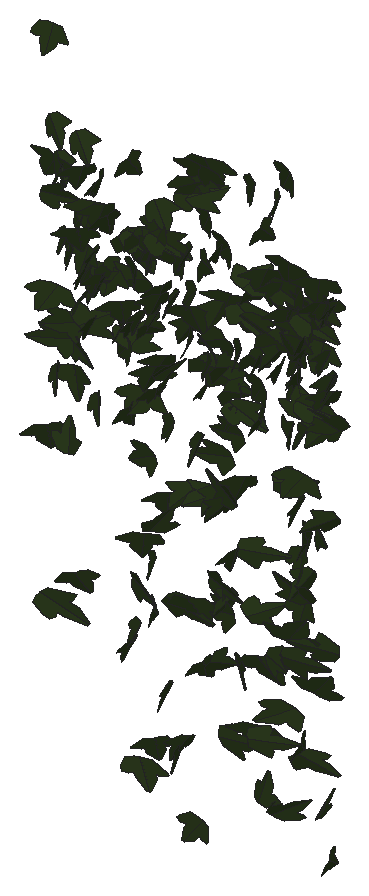
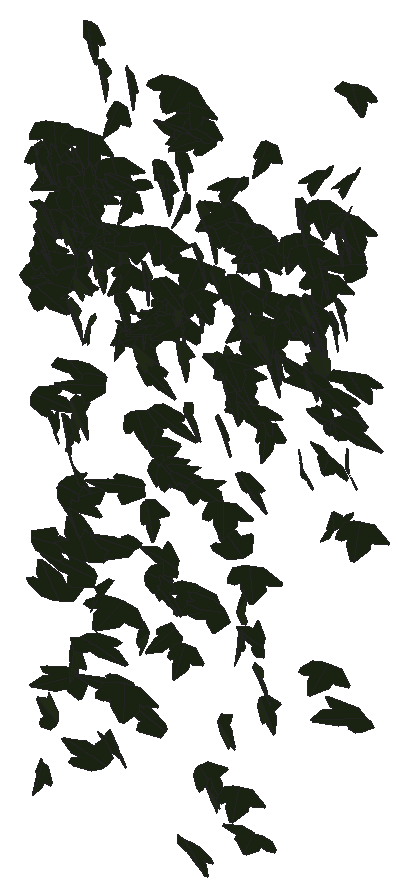
# SketchUp Ruby script. Lengths in millimetres.
U = 1.mm
M = Sketchup.active_model
def pt(a) = Geom::Point3d.new(a.map { |v| v * U })
def face(e, loops, mat)
  f = e.add_face(loops[0].map { |a| pt(a) })
  loops[1..].each { |l| e.add_face(l.map { |a| pt(a) }).erase! }
  f.material = f.back_material = mat if mat
  f
end
# faces: each face lists its corners as indices into pts; further lists are holes
def faces(e, pts, list, mat = nil) = list.each { |f| face(e, (f[0].is_a?(Array) ? f : [f]).map { |l| l.map { |i| pts[i] } }, mat) }
# xy, xz, yz: faces in a plane at the given z, y or x. An outline is a flat list of corners, or four numbers for a rectangle; further outlines are holes
def ring(l) = l.size == 4 ? [[l[0], l[1]], [l[2], l[1]], [l[2], l[3]], [l[0], l[3]]] : l.each_slice(2).to_a
def flat(e, list, mat, &to3) = list.each { |f| face(e, (f[0].is_a?(Array) ? f : [f]).map { |l| ring(l).map { |u, v| to3.(u, v) } }, mat) }
def xy(e, z, list, mat = nil) = flat(e, list, mat) { |x, y| [x, y, z] }
def xz(e, y, list, mat = nil) = flat(e, list, mat) { |x, z| [x, y, z] }
def yz(e, x, list, mat = nil) = flat(e, list, mat) { |y, z| [x, y, z] }
def lines(e, pts, list) = list.each { |a, b| e.add_line(pt(pts[a]), pt(pts[b])) }
# prism: a flat outline (further loops are holes) pulled along v
def prism(e, loops, v, mat = nil)
  f = face(e, loops, mat); d = Geom::Vector3d.new(v.map { |x| x * U })
  f.pushpull(f.normal.samedirection?(d) ? d.length : -d.length)
end
def box(e, o, s, mat = nil) = prism(e, [[o, [o[0] + s[0], o[1], o[2]], [o[0] + s[0], o[1] + s[1], o[2]], [o[0], o[1] + s[1], o[2]]]], [0, 0, s[2]], mat)
def at(x, y, z, deg = 0) = Geom::Transformation.translation(pt([x, y, z])) * Geom::Transformation.rotation(ORIGIN, Z_AXIS, deg.degrees)
def axes(o, x, y, z) = Geom::Transformation.new([*x, 0, *y, 0, *z, 0, *pt(o).to_a, 1])
def part(name) = M.definitions.add(name)
# library, detail: a bought-in or finely detailed component or shape, given as its bounding box
def library(name, o, s) = part(name).tap { |d| box(d.entities, o, s) }
def detail(e, o, s) = box(e.add_group.entities, o, s)
def put(e, d, t, mat = nil) = e.add_instance(d, t).tap { |i| i.material = mat if mat }
def group(e, t, mat = nil) = e.add_group.tap { |g| g.transformation = t; g.material = mat if mat }.entities
root = M.entities
M.materials.add("efeu2").color = [43, 57, 29]
c1 = part("ivyleaf_10")
p = [[0,12.8,-0.8],[-1.5,51.3,-10.9],[-4.9,51,-11.6],[-13.6,26.5,-7.3],[-13.2,15.9,-4.6],[-21.1,19.3,-7.2],
  [-29.5,16.3,-8.3],[-29.2,8.3,-6.2],[-19.7,-9.8,0.5],[-7.6,-13,4],[1,-12.2,5.8],[-0.4,51.1,-11.1],
  [-1.5,51.1,-10.9],[1,-12.4,5.9],[16.9,-12.4,3.5],[35.1,9.1,-5.1],[35,12.9,-6.1],[20.5,16.4,-4.9],
  [15.8,15,-3.8],[15.3,27.6,-7.1],[12.8,31.3,-7.8]]
faces(c1.entities,p,[[0,1,2,3,4,5,6,7,8,9,10],[11,12,0,13,14,15,16,17,18,19,20]],"efeu2")
put(root,c1,axes([857.1,1048,494],[-0.76417,-0.56364,-0.16539],[0.1854,0.13367,-0.69203],[1.10248,-0.41316,0.00174]))
put(root,c1,axes([875.9,1057.8,630.2],[0.62914,-0.04984,-0.57145],[-1.07511,0.08633,-0.3343],[0.18971,0.65451,0.00058]))
put(root,c1,axes([856.2,1056.8,1082.8],[0.86369,0.09119,-0.06828],[-0.08573,0.01132,-0.71351],[-0.10938,0.71114,0.02012]))
put(root,c1,axes([872.4,1048.6,897.9],[-1.16361,0.05516,0.27789],[-0.53203,-0.01005,-0.61304],[-0.08762,-0.67151,0.032]))
put(root,c1,axes([862.5,1054.4,698],[1.15679,0.14069,-0.19865],[-0.37438,-0.03088,-0.62374],[-0.27291,0.63871,0.0136]))
put(root,c1,axes([862.7,1060,578.1],[0.46837,-0.34978,0.49712],[0.59384,-0.38757,-0.42716],[0.99279,0.39684,0.02098]))
put(root,c1,axes([875.6,1051.7,887.6],[0.36125,-0.62169,-0.15977],[-0.00089,0.16647,-0.64834],[1.22165,0.18396,0.04677]))
put(root,c1,axes([871.3,1044.2,956.8],[0.07417,0.6859,-0.01278],[-0.00011,-0.01279,-0.68701],[-1.30563,0.03897,-0.00067]))
put(root,c1,axes([891.2,1053.3,661.6],[0.80097,-0.16994,-0.48499],[-0.85913,0.17735,-0.45386],[0.46745,0.61716,-0.00312]))
put(root,c1,axes([862.4,1046.6,844.8],[0.22257,-0.09676,0.68328],[0.60747,0.5078,-0.06104],[-0.58293,0.49224,0.19728]))
put(root,c1,axes([879.6,1055.6,783],[0.43516,-0.59083,-0.12994],[-0.02273,0.13448,-0.63247],[1.15111,0.22601,0.03663]))
put(root,c1,axes([883.5,1054.5,881.1],[0.46084,-0.57742,-0.21843],[-0.01855,0.23103,-0.62152],[1.1748,0.23015,0.07587]))
put(root,c1,axes([879.2,1048,902.4],[0.0145,0.67002,-0.10036],[-0.00753,-0.10032,-0.67006],[-1.28939,0.00812,0.00278]))
put(root,c1,axes([889.4,1054.8,764.6],[0.41365,-0.53615,-0.27461],[-0.06271,0.28092,-0.57454],[1.14473,0.20913,0.06776]))
put(root,c1,axes([864.2,1046,242.4],[0.609,0.20168,0.61131],[1.00332,0.30965,-0.37811],[-0.70305,0.61661,-0.01007]))
put(root,c1,axes([894.2,1044.3,482.4],[0.22662,0.60555,-0.37945],[0.10475,0.37577,0.61695],[1.35602,-0.13023,0.01576]))
put(root,c1,axes([890.1,1061.3,582.8],[1.0221,-0.25445,0.29182],[0.52582,-0.09774,-0.59366],[0.51623,0.60334,0.0269]))
put(root,c1,axes([906.6,1054.5,828.8],[0.49026,-0.5364,-0.28712],[-0.1041,0.29012,-0.59107],[1.15324,0.25422,0.06871]))
put(root,c1,axes([906.8,1050.1,291.4],[-0.81787,-0.39488,-0.26374],[0.33783,0.19634,-0.58319],[0.83824,-0.46442,-0.0223]))
put(root,c1,axes([911.5,1045.7,805.6],[-0.88124,-0.45718,-0.09759],[0.11767,0.07626,-0.65061],[0.88189,-0.46702,-0.01071]))
put(root,c1,axes([913.5,1054.2,746.1],[0.28575,-0.62987,-0.03437],[-0.0113,0.03391,-0.64751],[1.2005,0.15024,0.00209]))
put(root,c1,axes([916,1046.3,899.7],[-0.52099,-0.60983,-0.01375],[0.00795,0.0132,-0.66845],[1.16089,-0.27377,-0.00159]))
put(root,c1,axes([907.1,1054.1,696.2],[-0.00905,-0.59614,-0.30589],[0.16466,-0.30388,0.59089],[-1.26454,-0.0353,0.07913]))
put(root,c1,axes([895.3,1055.6,628.7],[0.19219,-0.14159,0.61257],[1.06825,-0.25923,-0.15244],[0.53911,0.56413,0.08369]))
put(root,c1,axes([918.4,1053.9,750.5],[0.5931,-0.52045,-0.23254],[-0.09072,0.2403,-0.6017],[1.08109,0.30569,0.07708]))
put(root,c1,axes([913.6,1056,773.9],[1.02959,-0.36291,0.04755],[0.09164,-0.01356,-0.65125],[0.69055,0.5429,0.01552]))
put(root,c1,axes([915.3,1044.1,946.2],[0.22831,0.67336,0.03139],[0.02708,0.02935,-0.68391],[-1.28265,0.12048,-0.00885]))
put(root,c1,axes([925.9,1056.9,843.2],[-0.82751,-0.47216,0.13175],[0.03176,-0.19027,-0.62679],[0.9324,-0.41256,0.13828]))
put(root,c1,axes([926,1060.1,773.5],[0.27136,-0.62096,0.10312],[0.0211,-0.10324,-0.637],[1.19781,0.1425,-0.01214]))
put(root,c1,axes([930.7,1049.1,679.8],[0.12703,-0.64604,-0.0109],[0.00227,0.01108,-0.64947],[1.22972,0.06672,0.00233]))
put(root,c1,axes([930.7,1052,737.8],[0.64574,-0.54433,0.07814],[0.15255,-0.04188,-0.6398],[1.03541,0.34564,0.04553]))
put(root,c1,axes([938,1052.8,887.7],[0.06274,-0.63429,-0.20279],[-0.0046,0.20292,-0.6351],[1.26736,0.03213,0.00773]))
put(root,c1,axes([918.1,1054.4,669.9],[0.96753,-0.03834,-0.44472],[0.84925,0.02623,0.50783],[-0.02195,-0.67493,0.045]))
put(root,c1,axes([927.8,1062.1,555.7],[0.54519,-0.32214,0.46975],[0.62388,-0.33676,-0.43085],[0.88653,0.4351,0.01432]))
put(root,c1,axes([942.8,1050.6,893.3],[0.1952,-0.63779,-0.1852],[0.00244,0.18759,-0.6453],[1.26399,0.09813,0.02984]))
put(root,c1,axes([944.6,1052.9,848.4],[-0.45012,-0.61153,0.09292],[0.03054,-0.10552,-0.65356],[1.17682,-0.23116,0.0525]))
put(root,c1,axes([944.6,1049.2,748.5],[-0.22325,-0.63702,0.03551],[0.04043,-0.03998,-0.64712],[1.21358,-0.11585,0.02809]))
put(root,c1,axes([949.9,1058.6,754.7],[1.2012,-0.14606,0.04699],[0.0896,-0.00498,-0.6478],[0.27792,0.63288,0.00574]))
put(root,c1,axes([956.5,1049.5,840.2],[-0.3484,-0.58618,-0.2297],[0.12459,0.22019,-0.61409],[1.19172,-0.19439,-0.00295]))
put(root,c1,axes([951.5,1052.6,765.3],[-0.27304,-0.46592,-0.42649],[0.47373,0.36026,-0.4773],[1.10487,-0.26961,0.09925]))
put(root,c1,axes([977.8,1049.6,687.5],[0.27409,-0.58308,-0.26247],[-0.03374,0.26531,-0.59909],[1.21649,0.13873,0.04252]))
put(root,c1,axes([997.3,1061.9,759],[-0.62477,-0.09847,0.53734],[-0.90721,-0.25459,-0.33787],[0.50787,-0.57592,0.05748]))
put(root,c1,axes([981.1,1047.7,720.1],[-0.7508,-0.48964,-0.10766],[0.13887,0.07946,-0.62875],[0.94399,-0.40113,0.00687]))
put(root,c1,axes([991.2,1043.9,667.4],[0.67988,-0.47449,-0.34447],[-0.19166,0.34772,-0.58341],[1.09936,0.35406,0.11132]))
put(root,c1,axes([990.8,1056.4,218.1],[0.0504,-0.6428,0.04508],[0.00002,-0.04512,-0.64335],[1.22639,0.02642,-0.00184]))
put(root,c1,axes([997.9,1042.3,574.3],[-0.19252,-0.62725,-0.29772],[0.1593,0.28766,-0.63447],[1.31179,-0.12699,0.03335]))
put(root,c1,axes([1000.1,1048.8,702.5],[0.07692,-0.64841,-0.01327],[-0.00157,0.01325,-0.64967],[1.23431,0.04043,0]))
put(root,c1,axes([999.6,1048.4,780.5],[0.5806,-0.48239,-0.29893],[-0.00711,0.33767,-0.54871],[1.08005,0.26154,0.15709]))
put(root,c1,axes([989.3,1048,823.4],[-0.49488,-0.289,-0.60205],[0.84834,0.406,-0.3874],[0.94645,-0.51502,0.03244]))
put(root,c1,axes([1000,1040,945.6],[-0.1955,-0.55324,-0.38747],[0.31397,0.3595,-0.55705],[1.24655,-0.17731,0.07954]))
put(root,c1,axes([1005.2,1049,249.9],[0.52143,-0.59078,0.0055],[0.00324,-0.00527,-0.65121],[1.12441,0.27398,-0.00067]))
put(root,c1,axes([1019.4,1055.3,506.3],[0.69284,-0.33146,-0.44071],[-0.56009,0.32981,-0.49115],[0.88756,0.46687,0.03408]))
put(root,c1,axes([1012.4,1056.1,818.8],[0.50962,-0.58215,-0.12562],[-0.10595,0.11266,-0.64077],[1.12848,0.27347,-0.00343]))
put(root,c1,axes([1004.9,1055.2,812.5],[-1.17968,-0.09076,-0.18297],[0.37808,-0.13209,-0.60746],[0.09031,-0.63264,0.15308]))
put(root,c1,axes([1011.2,1052.7,716.2],[0.02976,-0.62675,0.13313],[0.0523,-0.13239,-0.6265],[1.21831,0.02099,0.02364]))
put(root,c1,axes([1014,1054.1,383.8],[-0.87919,-0.46919,0.00578],[-0.0018,-0.00717,-0.65843],[0.89304,-0.46193,0.00436]))
put(root,c1,axes([999.6,1047.3,670.7],[0.93123,0.35894,-0.34003],[0.52847,0.19633,0.60681],[0.77858,-0.56257,-0.00518]))
put(root,c1,axes([992.4,1064,303.4],[0.02802,-0.12796,0.64505],[1.10604,-0.29945,-0.07267],[0.58578,0.57152,0.10635]))
put(root,c1,axes([1016.6,1048.7,598.8],[1.16993,0.12094,-0.20602],[-0.38777,-0.03154,-0.62645],[-0.23739,0.64756,0.00797]))
put(root,c1,axes([1009.2,1043.6,833.8],[-0.31597,-0.43543,-0.47158],[0.47115,0.40598,-0.46201],[1.12708,-0.29178,0.06092]))
put(root,c1,axes([1004.8,1059.7,40.6],[1.14469,0.08302,0.1919],[0.36205,0.02524,-0.60716],[-0.16514,0.63082,-0.00097]))
put(root,c1,axes([1037.2,1048,825.6],[-1.13481,-0.15913,0.3482],[-0.63875,-0.09279,-0.61713],[0.35054,-0.68422,0.00271]))
put(root,c1,axes([1006.7,1046,832],[0.70892,0.3458,0.47277],[0.57403,0.36705,-0.50611],[-0.95563,0.47701,0.04671]))
put(root,c1,axes([1019.7,1059.9,809.9],[-0.1092,0.38291,-0.5213],[0.01877,-0.52277,-0.38507],[-1.23089,-0.04194,0.04038]))
put(root,c1,axes([1015.3,1069.4,341.7],[0.08738,-0.0821,0.63986],[0.59469,-0.55838,-0.09406],[1.07414,0.31582,0.00003]))
put(root,c1,axes([1031.6,1051.3,639.4],[-0.45159,-0.60961,0.11718],[-0.03064,-0.11937,-0.65357],[1.18106,-0.23619,0.02785]))
put(root,c1,axes([1028.8,1044.6,813.9],[0.51601,-0.54341,-0.23966],[-0.01518,0.2601,-0.59877],[1.13022,0.25159,0.10138]))
put(root,c1,axes([1030.7,1055.4,85.7],[-0.70846,-0.50574,-0.14921],[0.19503,0.10978,-0.62774],[0.98442,-0.38572,0.01698]))
put(root,c1,axes([1033,1054.5,724.5],[0.3373,-0.61623,-0.05313],[-0.034,0.05015,-0.6412],[1.17667,0.1781,-0.0033]))
put(root,c1,axes([1027.6,1043.5,709.6],[-0.25734,-0.34351,-0.52703],[0.36256,0.4914,-0.36916],[1.14108,-0.2336,-0.00156]))
put(root,c1,axes([1035.1,1051.1,611.3],[-0.26087,-0.61505,-0.13798],[0.06663,0.13356,-0.63012],[1.1978,-0.14138,0.005]))
put(root,c1,axes([1034.1,1046.5,288.3],[0.24512,-0.42891,-0.45533],[0.0605,0.46877,-0.43258],[1.18897,0.06457,0.11588]))
put(root,c1,axes([1040.3,1049,751.2],[-0.35784,-0.62016,0.0716],[-0.01885,-0.0718,-0.64794],[1.18798,-0.18794,0.01129]))
put(root,c1,axes([1041.3,1058.9,656.3],[-0.48529,-0.57901,0.11083],[-0.065,-0.10604,-0.63257],[1.12009,-0.25702,0.01131]))
put(root,c1,axes([1039.9,1057.5,762],[-0.2828,-0.62434,-0.05258],[0.01644,0.05199,-0.64177],[1.19234,-0.1488,-0.00362]))
put(root,c1,axes([1038.6,1048.7,858.2],[0.937,-0.41894,-0.11947],[-0.08803,0.129,-0.64295],[0.82442,0.48992,0.06713]))
put(root,c1,axes([1035.7,1051.6,407.1],[-0.40572,-0.60311,0.18181],[0.12831,0.169,0.63963],[-1.19197,0.22347,0.00697]))
put(root,c1,axes([1043.2,1045.5,889.2],[0.40141,0.64012,0.1146],[0.00193,0.12015,-0.673],[-1.23765,0.2078,0.03612]))
put(root,c1,axes([1051.5,1056.3,457],[-0.74392,-0.51791,-0.06961],[0.06998,0.05945,-0.64883],[0.99209,-0.39255,-0.00643]))
put(root,c1,axes([1051,1056.9,637.3],[0.25722,-0.61537,-0.1097],[-0.00233,0.11197,-0.62964],[1.18964,0.13328,0.02248]))
put(root,c1,axes([1049.1,1059.6,170.4],[0.33309,-0.581,0.25946],[0.16491,-0.24482,-0.60668],[1.19972,0.19496,0.01136]))
put(root,c1,axes([1056.1,1054.9,566.6],[0.48991,-0.54775,-0.2026],[-0.11912,0.19426,-0.60472],[1.10511,0.26376,0.02463]))
put(root,c1,axes([1049.5,1046.2,641.6],[0.14587,-0.44703,0.44825],[0.14728,0.45475,0.44028],[-1.19579,0.00148,0.10891]))
put(root,c1,axes([1063,1054.8,758.5],[0.37693,-0.60292,0.15583],[0.06213,-0.15325,-0.6344],[1.18355,0.20006,-0.01633]))
put(root,c1,axes([1046.4,1043.9,843],[0.63559,0.29565,0.55088],[0.57234,0.47159,-0.4354],[-1.04319,0.43887,0.09675]))
put(root,c1,axes([1063.2,1064.4,82.3],[0.37095,-0.51288,0.32323],[0.28599,-0.28806,-0.54768],[1.11778,0.24391,0.03286]))
put(root,c1,axes([1075.6,1061.2,101.2],[-0.21543,-0.60518,0.21047],[-0.07186,-0.20706,-0.61567],[1.21732,-0.11932,0.0009]))
put(root,c1,axes([1073.5,1053.9,817.5],[0.66072,-0.50532,-0.24475],[-0.08834,0.26095,-0.60459],[1.06493,0.33516,0.1017]))
put(root,c1,axes([1085.2,1060,475.6],[-0.52438,-0.35239,0.45368],[-0.1162,-0.48235,-0.41173],[1.08711,-0.22154,0.17483]))
put(root,c1,axes([1087.5,1062.2,725.7],[-0.39235,-0.5524,0.24581],[-0.06907,-0.24793,-0.58761],[1.14865,-0.2036,0.04863]))
put(root,c1,axes([1087.6,1051.4,836.1],[0.39834,-0.63045,0.02736],[0.01022,-0.02704,-0.66427],[1.20095,0.20934,-0.00342]))
put(root,c1,axes([1096.6,1049.1,779.4],[0.41164,-0.56569,-0.2598],[-0.15802,0.24636,-0.60555],[1.17415,0.23148,0.00958]))
put(root,c1,axes([1072.9,1047.7,310.9],[-0.54109,0.07812,-0.60434],[1.11882,-0.14041,-0.29471],[-0.30534,-0.65294,-0.00893]))
put(root,c1,axes([1098.9,1041.8,714.6],[0.24233,-0.57756,-0.38663],[-0.08657,0.3853,-0.59055],[1.31993,0.13131,0.03225]))
put(root,c1,axes([1103.6,1052.3,-10.5],[0.99754,-0.33783,-0.14401],[-0.23327,0.07566,-0.62357],[0.65886,0.53827,-0.00273]))
put(root,c1,axes([1101.5,1044.5,755.2],[-1.15905,-0.27487,-0.13611],[0.23906,0.05254,-0.66815],[0.53256,-0.62181,0.00371]))
put(root,c1,axes([1094.1,1037.6,927.7],[0.28563,0.12887,0.69477],[0.24341,0.69359,-0.15627],[-1.32264,0.15547,0.12128]))
put(root,c1,axes([1102.1,1043.7,322.6],[-1.19853,-0.1172,-0.22907],[0.42706,0.04626,-0.64054],[0.23967,-0.66851,-0.00417]))
put(root,c1,axes([1104.5,1053.6,560.2],[0.57734,-0.60504,0.24995],[0.20011,-0.22688,-0.67679],[1.22974,0.32098,-0.00722]))
put(root,c1,axes([1114.9,1044.9,970.6],[-1.28249,0.01628,0.13224],[-0.25181,-0.00125,-0.67404],[-0.02994,-0.68671,0.00436]))
put(root,c1,axes([1103.4,1046,948.4],[-1.02542,-0.3581,-0.20826],[0.42649,0.03542,-0.64065],[0.6631,-0.57655,0.08999]))
put(root,c1,axes([1123.6,1060.5,483.1],[-0.63386,-0.14414,0.53416],[-0.46752,-0.52013,-0.29351],[0.9435,-0.35456,0.21342]))
put(root,c1,axes([1115.1,1054.7,645.7],[0.11798,-0.60669,-0.21449],[-0.04838,0.21301,-0.60984],[1.22374,0.06691,-0.00343]))
put(root,c1,axes([1119,1050.9,898.7],[0.71585,-0.4555,-0.31889],[-0.0872,0.3583,-0.56583],[1.05464,0.3388,0.16967]))
put(root,c1,axes([1120.9,1043.2,238.5],[-0.39077,-0.52572,-0.32906],[0.22798,0.30648,-0.5644],[1.15817,-0.23771,0.00007]))
put(root,c1,axes([1140.3,1055.9,722],[-0.76835,0.1312,0.47502],[-0.9187,0.01837,-0.41533],[-0.18886,-0.62313,0.08777]))
put(root,c1,axes([1102,1046.3,926.3],[0.78752,0.00326,-0.54265],[0.96293,0.2444,0.38728],[0.37339,-0.63715,0.14577]))
put(root,c1,axes([1125.7,1046.1,685],[0.41127,-0.56641,-0.23081],[-0.06946,0.23242,-0.60452],[1.16199,0.21437,0.04555]))
put(root,c1,axes([1120.7,1040.9,836.2],[0.21785,-0.4952,-0.43868],[0.26551,0.45325,-0.47525],[1.23077,-0.01013,0.18017]))
put(root,c1,axes([1113.9,1054.8,680.8],[-0.71866,-0.27584,-0.44025],[0.75271,0.20029,-0.46471],[0.64114,-0.54432,0.0521]))
put(root,c1,axes([1127.4,1065.9,486.5],[-0.19258,-0.56434,0.41807],[0.08605,-0.42674,-0.56511],[1.3339,-0.05395,0.09681]))
put(root,c1,axes([1131.9,1045,704.2],[0.61077,-0.12287,-0.5951],[-0.26232,0.64074,-0.20662],[1.12634,0.21585,0.27458]))
put(root,c1,axes([1144.2,1054.5,550.7],[0.58588,-0.14818,-0.54839],[-0.95117,0.22584,-0.34158],[0.5139,0.58693,-0.00702]))
put(root,c1,axes([1128.5,1044.2,985.8],[-1.29166,-0.06143,-0.11158],[0.21229,0.00544,-0.68144],[0.11704,-0.68777,0.00458]))
put(root,c1,axes([1137.8,1054.8,857.7],[0.12583,-0.62024,-0.20868],[0.01048,0.21026,-0.6232],[1.24542,0.0609,0.02633]))
put(root,c1,axes([1140.5,1054.6,771.1],[-0.43121,-0.5453,0.26649],[0.04299,-0.29184,-0.57795],[1.15432,-0.19284,0.12108]))
put(root,c1,axes([1152.5,1052.1,321.1],[0.48989,-0.27645,-0.58411],[-0.72807,0.44155,-0.37756],[0.99124,0.46095,0.01136]))
put(root,c1,axes([1146,1055.5,480.5],[-0.24993,-0.53477,0.34231],[-0.13661,-0.33481,-0.55059],[1.20068,-0.14941,0.00861]))
put(root,c1,axes([1163.9,1043,497.7],[-0.56081,0.27244,-0.56884],[-0.77557,0.39697,0.40122],[0.91617,0.50281,-0.00855]))
put(root,c1,axes([1153.6,1057,787.8],[-1.0793,-0.28892,0.10619],[-0.17028,-0.05827,-0.63636],[0.56055,-0.574,0.01115]))
put(root,c1,axes([1149.4,1064.6,338.4],[-0.09106,-0.32684,0.54806],[0.12901,-0.54909,-0.32154],[1.20759,0.03402,0.07568]))
put(root,c1,axes([1155.2,1045.2,868.6],[0.67015,-0.34793,-0.46763],[-0.29031,0.47228,-0.46626],[1.07065,0.34585,0.16627]))
put(root,c1,axes([1143.6,1038.8,251.8],[-0.23864,-0.28147,-0.60718],[0.46669,0.55546,-0.30813],[1.18514,-0.27541,-0.00092]))
put(root,c1,axes([1129.6,1055.9,356.6],[-0.02131,-0.09365,0.63728],[1.18364,-0.16748,-0.01369],[0.3191,0.61498,0.09332]))
put(root,c1,axes([1146.8,1044.4,688.9],[-0.22171,-0.28765,-0.66456],[0.48137,0.61455,-0.31034],[1.2914,-0.27846,0.00158]))
put(root,c1,axes([1171.1,1046.7,596.5],[0.50372,-0.15479,-0.55967],[-0.80555,0.36966,-0.3024],[0.75661,0.49662,0.05065]))
put(root,c1,axes([1144.1,1051.5,672.6],[-0.6986,-0.23463,-0.47744],[0.85629,0.17258,-0.43072],[0.54022,-0.57698,0.06531]))
put(root,c1,axes([1165.3,1051.7,415.6],[-0.13228,-0.67732,-0.12922],[0.0344,0.12804,-0.68086],[1.31187,-0.07166,0.00482]))
put(root,c1,axes([1170.5,1060.7,629.8],[0.17206,-0.53137,0.45675],[0.13659,-0.45109,-0.53899],[1.32655,0.11537,-0.00374]))
put(root,c1,axes([1165.9,1039.9,661.9],[-0.27943,-0.2353,-0.60205],[0.58096,0.51896,-0.27727],[1.0844,-0.33866,-0.00659]))
put(root,c1,axes([1167.4,1058.4,252],[-0.39987,0.48136,-0.37522],[0.20806,-0.36073,-0.52399],[-1.14279,-0.23411,0.03589]))
put(root,c1,axes([1179.3,1044.5,660],[0.30728,-0.43353,-0.48199],[-0.10447,0.48579,-0.45534],[1.22938,0.14964,0.08178]))
put(root,c1,axes([1179,1041.4,723.1],[0.37229,-0.59786,-0.34202],[-0.04927,0.34891,-0.62472],[1.30996,0.18304,0.0737]))
put(root,c1,axes([1181.5,1049.5,529.1],[-0.54952,-0.58596,0.0746],[-0.0453,-0.07142,-0.65316],[1.12328,-0.28954,0.01015]))
put(root,c1,axes([1154.4,1053.9,134.4],[0.39072,-0.1159,-0.63974],[1.04137,-0.33154,0.23565],[-0.66831,-0.58437,-0.00681]))
put(root,c1,axes([1174.2,1057.4,775.4],[0.92563,0.23696,0.35419],[0.61987,0.13991,-0.54082],[-0.52303,0.58517,-0.01412]))
put(root,c1,axes([1200,1055.9,162.9],[-1.17534,-0.32765,0.00284],[-0.00446,-0.00163,-0.6991],[0.62359,-0.61757,0.00034]))
put(root,c1,axes([1194.5,1049.8,817.5],[-0.13498,-0.46994,-0.45003],[0.2217,0.43622,-0.47387],[1.21836,-0.13144,0.03637]))
put(root,c1,axes([1178.2,1041.1,638.5],[0.60304,0.32075,0.47654],[0.65517,0.32965,-0.45077],[-0.87521,0.46778,-0.00909]))
put(root,c1,axes([1199.1,1045,975.1],[0.57678,-0.56381,-0.24768],[-0.01071,0.2735,-0.62948],[1.17197,0.27998,0.11614]))
put(root,c1,axes([1195.5,1050.5,718.5],[-0.36371,-0.41764,-0.47317],[0.43433,0.4152,-0.45864],[1.11986,-0.29667,0.0242]))
put(root,c1,axes([1187.7,1057.5,765.6],[-0.72835,0.09507,-0.52218],[0.97981,-0.09013,-0.39371],[-0.24575,-0.6411,-0.02209]))
put(root,c1,axes([1194.2,1044.5,829],[0.83481,0.21179,-0.47557],[0.60297,0.38486,0.46361],[0.78621,-0.52005,0.14941]))
put(root,c1,axes([1210.1,1047.6,678.6],[0.78458,-0.44987,-0.32144],[-0.16232,0.34442,-0.5914],[1.0397,0.39325,0.15023]))
put(root,c1,axes([1211.3,1044.5,632.1],[-0.03727,-0.46523,-0.47929],[0.08301,0.47758,-0.46535],[1.26853,-0.04492,0.01637]))
put(root,c1,axes([1215,1039.7,730],[0.17974,-0.52721,-0.47273],[-0.01387,0.47617,-0.5325],[1.34762,0.07522,0.05757]))
put(root,c1,axes([1220.1,1048.3,850.8],[-0.68771,-0.54866,0.07499],[-0.04763,-0.07327,-0.65667],[1.05283,-0.36169,0.01927]))
put(root,c1,axes([1194.4,1046,431.8],[0.01975,-0.08525,-0.65903],[1.16483,0.25796,-0.02374],[0.49262,-0.60654,0.08254]))
put(root,c1,axes([1212,1053.3,269.8],[-1.1684,-0.21507,-0.27299],[0.48852,0.09296,-0.65049],[0.4459,-0.66541,-0.00264]))
put(root,c1,axes([1215.5,1048.4,71.4],[0.97371,-0.44222,0.07315],[-0.09167,0.05612,0.67616],[-0.84812,-0.51376,0.01089]))
put(root,c1,axes([1220.1,1040.8,920.9],[-0.14211,-0.50124,-0.45425],[0.29162,0.43259,-0.50254],[1.25396,-0.15741,0.06539]))
put(root,c1,axes([1207.3,1040.6,344.7],[0.42754,0.16439,-0.57322],[0.85324,0.35734,0.27818],[0.74835,-0.50135,0.01032]))
put(root,c1,axes([1232.2,1056.4,736.4],[-0.05441,-0.46082,0.44097],[0.01916,-0.44168,-0.46091],[1.21374,-0.01368,0.02705]))
put(root,c1,axes([1212.2,1042.7,157.8],[0.17988,-0.04771,-0.64398],[1.18699,0.17544,0.07854],[0.31855,-0.62679,0.071]))
put(root,c1,axes([1239.9,1052.8,837.2],[-0.46299,-0.61296,0.06258],[-0.03066,-0.06093,-0.65943],[1.17226,-0.24369,0.00747]))
put(root,c1,axes([1234.6,1043.6,285.3],[-0.17357,0.49591,0.41119],[-0.13315,0.40521,-0.50421],[-1.2188,-0.11489,-0.00348]))
put(root,c1,axes([1238.9,1054.3,717.7],[0.09487,-0.63913,-0.08309],[0.01758,0.08404,-0.64088],[1.2265,0.04823,0.01562]))
put(root,c1,axes([1229.8,1048.8,760.7],[-0.6525,-0.36394,-0.40618],[0.63932,0.23705,-0.49593],[0.8177,-0.47575,0.06362]))
put(root,c1,axes([1241.7,1043.6,970],[0.29579,-0.63244,-0.21257],[0.00335,0.21865,-0.64923],[1.26982,0.14674,0.05123]))
put(root,c1,axes([1252.3,1051.8,210],[0.87157,0.12814,-0.46823],[-0.86106,-0.1207,-0.47552],[-0.33494,0.64373,0.00404]))
put(root,c1,axes([1252.9,1051.3,802.5],[-0.60241,-0.58238,-0.04341],[0.03214,0.04023,-0.66282],[1.111,-0.31694,-0.00436]))
put(root,c1,axes([1259.3,1050.4,873.7],[-1.24175,0.09455,0.1204],[-0.23204,-0.00217,-0.65898],[-0.1762,-0.66346,0.01931]))
put(root,c1,axes([1257.2,1045.8,626.2],[0.22012,-0.09608,-0.65701],[-0.03255,0.66625,-0.10044],[1.2633,0.03391,0.11189]))
put(root,c1,axes([1243.9,1051.2,55.7],[-0.35437,-0.46109,0.44643],[0.42112,0.39022,0.49532],[-1.14658,0.28583,0.04394]))
put(root,c1,axes([1274.2,1055.5,796.6],[-0.92694,-0.08585,0.43355],[-0.81197,-0.07713,-0.49455],[0.21964,-0.64747,0.00143]))
put(root,c1,axes([1263.6,1052.7,829.3],[-1.17314,0.22371,0.13248],[-0.25871,0.01328,-0.6549],[-0.4218,-0.63034,0.03322]))
put(root,c1,axes([1260.3,1041.6,1014],[0.79145,-0.43477,-0.3496],[-0.1399,0.38953,-0.57187],[1.05253,0.3787,0.18687]))
put(root,c1,axes([1257.9,1065.5,693.6],[0.14784,-0.49211,0.4212],[0.22521,-0.4063,-0.49652],[1.21206,0.13552,0.04088]))
put(root,c1,axes([1279.1,1050.2,389.2],[-0.87393,0.08336,-0.43854],[-0.82871,0.05495,0.46637],[0.18715,0.63258,0.01728]))
put(root,c1,axes([1255.8,1052.8,762.6],[-1.09158,0.20995,-0.23148],[0.36758,-0.14221,-0.60753],[-0.46759,-0.60193,0.0628]))
put(root,c1,axes([1238.6,1050,834.8],[0.54966,0.03466,0.60123],[1.11367,0.14148,-0.28924],[-0.27096,0.65182,0.03081]))
put(root,c1,axes([1247,1049.2,550.4],[0.09037,-0.04763,-0.65548],[0.92492,0.44496,0.00287],[0.84204,-0.48365,0.06719]))
put(root,c1,axes([1264.9,1062.2,519.6],[0.28357,-0.71611,0.08053],[0.04243,-0.07761,-0.73142],[1.37084,0.15053,0.00598]))
put(root,c1,axes([1262.5,1049.4,323.6],[-1.24979,-0.2154,0.2012],[0.36802,0.05598,0.69107],[-0.42338,0.68452,0.0068]))
put(root,c1,axes([1271.3,1044.7,739.7],[0.48263,-0.56911,-0.22876],[-0.10457,0.22547,-0.62183],[1.16266,0.25652,0.03903]))
put(root,c1,axes([1269,1051.4,716.9],[0.0542,-0.5821,-0.28606],[0.10107,0.28747,-0.57968],[1.23026,0.00203,0.06022]))
put(root,c1,axes([1261,1067.2,440.7],[0.83711,-0.42576,0.38493],[0.49737,-0.28322,-0.61188],[0.97258,0.51129,-0.0184]))
put(root,c1,axes([1272.9,1046.3,842.4],[0.82169,-0.46357,-0.22263],[-0.11547,0.24274,-0.6231],[0.9719,0.42076,0.11419]))
put(root,c1,axes([1276.6,1048,564.9],[1.17412,0.0313,-0.20388],[-0.38749,-0.01063,-0.61771],[-0.06291,0.64965,-0.00028]))
put(root,c1,axes([1281.1,1054.5,787.2],[-1.08354,-0.31366,0.12038],[-0.147,-0.10832,-0.64754],[0.62229,-0.57174,0.05664]))
put(root,c1,axes([1275.3,1066.7,411.3],[-0.15414,-0.43169,0.57146],[0.15407,-0.57694,-0.42436],[1.35432,0.0165,0.11332]))
put(root,c1,axes([1279.1,1059,752.7],[0.06915,-0.66389,0.00621],[0.00265,-0.00614,-0.66488],[1.26357,0.03635,0.00106]))
put(root,c1,axes([1282.2,1047.8,637.8],[0.40519,-0.64095,-0.14218],[-0.10234,0.13194,-0.67532],[1.2453,0.21939,-0.00924]))
put(root,c1,axes([1275.4,1054.7,372.8],[1.00692,-0.37381,0.08968],[0.14678,-0.04624,-0.64777],[0.71675,0.53462,0.00667]))
put(root,c1,axes([1283,1045.6,777.1],[0.20314,-0.59206,-0.3014],[0.02191,0.30687,-0.59873],[1.26423,0.08981,0.05881]))
put(root,c1,axes([1285.8,1039,177.1],[-0.00969,-0.47896,-0.49731],[0.01547,0.49725,-0.47899],[1.31398,-0.00939,0.00197]))
put(root,c1,axes([1290.1,1049.9,485.9],[0.45079,-0.49707,-0.37628],[-0.11606,0.38212,-0.54317],[1.18083,0.22732,0.09027]))
put(root,c1,axes([1286.5,1045.7,668.5],[1.0973,0.28141,0.05878],[-0.11312,-0.0122,0.64139],[0.53532,-0.57941,0.01505]))
put(root,c1,axes([1290,1037.7,477.5],[0.05516,-0.34464,-0.53511],[0.00796,0.53575,-0.34482],[1.21133,0.01217,0.02664]))
put(root,c1,axes([1278.7,1053.8,806],[0.98298,-0.34605,0.23266],[0.46621,-0.04793,-0.61509],[0.64224,0.56444,0.09041]))
put(root,c1,axes([1264.8,1047.9,293.1],[0.15464,-0.00523,-0.64762],[1.19891,-0.15092,0.08025],[-0.28621,-0.63501,-0.01374]))
put(root,c1,axes([1282.9,1053,151],[-0.68673,-0.15428,-0.51251],[0.91854,0.17344,-0.392],[0.4404,-0.60232,0.01841]))
put(root,c1,axes([1318.7,1055.3,320.7],[0.0477,0.02157,0.63713],[-1.0138,-0.34957,0.03279],[0.66652,-0.53325,0.00428]))
put(root,c1,axes([1301,1053.6,826.1],[1.25488,-0.04096,-0.05098],[-0.08889,0.06659,-0.65758],[0.08711,0.65796,0.06338]))
put(root,c1,axes([1309.5,1048.3,867.3],[-0.99113,-0.41886,0.03252],[-0.01353,-0.043,-0.66769],[0.79947,-0.52001,0.02902]))
put(root,c1,axes([1291.1,1066.8,482.7],[-0.09678,0.05309,0.64855],[0.91895,-0.43302,0.07331],[0.83022,0.48549,-0.00554]))
put(root,c1,axes([1303.5,1058.2,764.3],[1.24015,-0.20335,0.02645],[0.04799,-0.00797,-0.68261],[0.38731,0.6521,-0.0001]))
put(root,c1,axes([1317.6,1059.4,513.6],[-0.20117,-0.3157,0.54538],[-0.33726,-0.51579,-0.33292],[1.15092,-0.20633,-0.00223]))
put(root,c1,axes([1312.5,1049.4,836.7],[-0.39955,-0.6397,-0.03572],[0.00983,0.0359,-0.67324],[1.21934,-0.2099,-0.00628]))
put(root,c1,axes([1289.8,1044.7,806.4],[0.63703,0.27444,0.5275],[0.7386,0.35781,-0.4324],[-0.85742,0.51212,0.01943]))
put(root,c1,axes([1303.1,1052.3,258.1],[-1.13003,-0.18347,0.21102],[0.39418,0.0442,0.62119],[-0.35754,0.62858,0.01791]))
put(root,c1,axes([1317.5,1055.9,650.5],[-0.55912,-0.41075,0.42034],[-0.20697,-0.42382,-0.49016],[1.0992,-0.28873,0.12152]))
put(root,c1,axes([1297.2,1035.9,687.5],[0.28623,0.31893,0.58519],[0.43584,0.53865,-0.35242],[-1.19117,0.27372,0.01167]))
put(root,c1,axes([1314.6,1050.2,840.4],[0.67571,-0.46871,-0.31687],[-0.16185,0.32563,-0.57696],[1.06455,0.34702,0.11341]))
put(root,c1,axes([1328.2,1052.7,659.1],[-0.76629,-0.17656,-0.50346],[-0.86953,-0.21161,0.43959],[-0.52435,0.60894,0.00679]))
put(root,c1,axes([1315.2,1058.1,759.8],[-0.05248,-0.61533,0.16209],[0.06187,-0.16339,-0.61474],[1.20946,-0.01834,0.03848]))
put(root,c1,axes([1321.6,1053.4,703],[-0.35277,-0.61522,0.17697],[-0.06318,-0.17475,-0.64229],[1.21673,-0.18745,0.01796]))
put(root,c1,axes([1318.5,1051.7,834.6],[-0.6958,-0.54994,-0.10257],[0.16046,0.06697,-0.65956],[1.05254,-0.37376,0.03275]))
put(root,c1,axes([1316.1,1044.1,83.8],[0.3111,-0.59471,0.29974],[-0.13908,0.29076,0.61673],[-1.25983,-0.17895,0.00593]))
put(root,c1,axes([1320.7,1053.6,724.5],[-0.15791,-0.61818,0.16046],[0.10584,-0.16819,-0.61919],[1.21089,-0.06592,0.07505]))
put(root,c1,axes([1324.7,1053.6,833.6],[0.19904,-0.6555,0.0077],[-0.03038,-0.01034,-0.66356],[1.24726,0.10436,-0.01739]))
put(root,c1,axes([1325.3,1050.1,13.9],[-0.03907,-0.38529,-0.50905],[0.0952,0.50678,-0.38559],[1.21131,-0.05226,0.01388]))
put(root,c1,axes([1326.5,1053.9,727.1],[0.42816,-0.60375,0.02625],[0.01881,-0.02433,-0.6443],[1.14998,0.22519,0.00076]))
